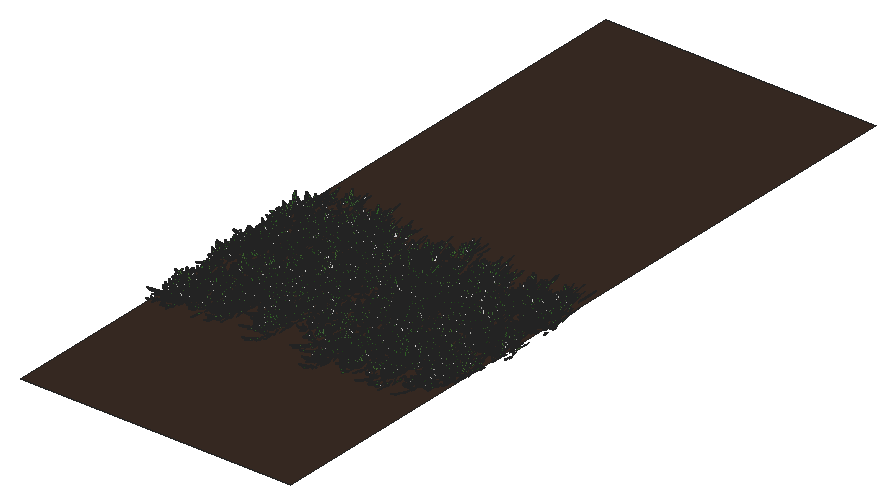
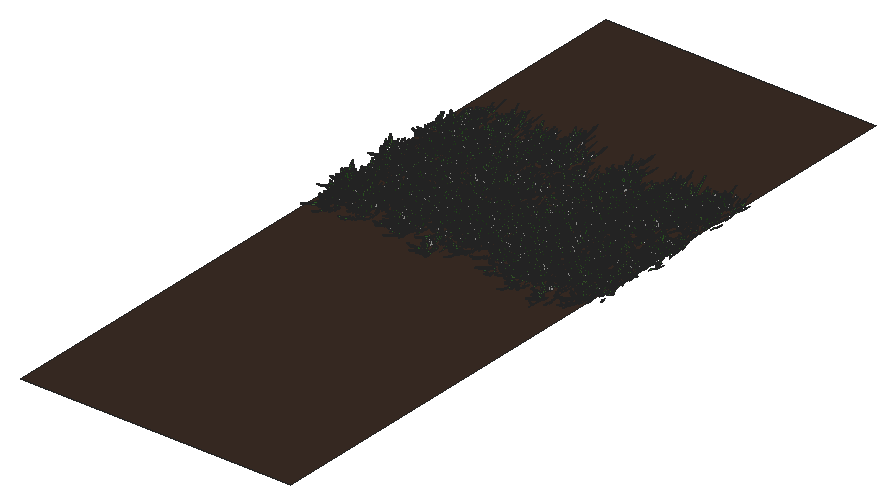
# SketchUp Ruby script. Lengths in inches.
U = 1.inch
M = Sketchup.active_model
def pt(a) = Geom::Point3d.new(a.map { |v| v * U })
def face(e, loops, mat)
  f = e.add_face(loops[0].map { |a| pt(a) })
  loops[1..].each { |l| e.add_face(l.map { |a| pt(a) }).erase! }
  f.material = f.back_material = mat if mat
  f
end
# faces: each face lists its corners as indices into pts; further lists are holes
def faces(e, pts, list, mat = nil) = list.each { |f| face(e, (f[0].is_a?(Array) ? f : [f]).map { |l| l.map { |i| pts[i] } }, mat) }
# xy, xz, yz: faces in a plane at the given z, y or x. An outline is a flat list of corners, or four numbers for a rectangle; further outlines are holes
def ring(l) = l.size == 4 ? [[l[0], l[1]], [l[2], l[1]], [l[2], l[3]], [l[0], l[3]]] : l.each_slice(2).to_a
def flat(e, list, mat, &to3) = list.each { |f| face(e, (f[0].is_a?(Array) ? f : [f]).map { |l| ring(l).map { |u, v| to3.(u, v) } }, mat) }
def xy(e, z, list, mat = nil) = flat(e, list, mat) { |x, y| [x, y, z] }
def xz(e, y, list, mat = nil) = flat(e, list, mat) { |x, z| [x, y, z] }
def yz(e, x, list, mat = nil) = flat(e, list, mat) { |y, z| [x, y, z] }
def lines(e, pts, list) = list.each { |a, b| e.add_line(pt(pts[a]), pt(pts[b])) }
# prism: a flat outline (further loops are holes) pulled along v
def prism(e, loops, v, mat = nil)
  f = face(e, loops, mat); d = Geom::Vector3d.new(v.map { |x| x * U })
  f.pushpull(f.normal.samedirection?(d) ? d.length : -d.length)
end
def box(e, o, s, mat = nil) = prism(e, [[o, [o[0] + s[0], o[1], o[2]], [o[0] + s[0], o[1] + s[1], o[2]], [o[0], o[1] + s[1], o[2]]]], [0, 0, s[2]], mat)
def at(x, y, z, deg = 0) = Geom::Transformation.translation(pt([x, y, z])) * Geom::Transformation.rotation(ORIGIN, Z_AXIS, deg.degrees)
def axes(o, x, y, z) = Geom::Transformation.new([*x, 0, *y, 0, *z, 0, *pt(o).to_a, 1])
def part(name) = M.definitions.add(name)
# library, detail: a bought-in or finely detailed component or shape, given as its bounding box
def library(name, o, s) = part(name).tap { |d| box(d.entities, o, s) }
def detail(e, o, s) = box(e.add_group.entities, o, s)
def put(e, d, t, mat = nil) = e.add_instance(d, t).tap { |i| i.material = mat if mat }
def group(e, t, mat = nil) = e.add_group.tap { |g| g.transformation = t; g.material = mat if mat }.entities
root = M.entities
M.materials.add("Material10").color = [48, 90, 38]
M.materials.add("Material11").color = [68, 110, 48]
M.materials.add("Material12").color = [48, 90, 48]
M.materials.add("Material13").color = [58, 110, 58]
M.materials.add("Material14").color = [58, 90, 38]
M.materials.add("Material15").color = [68, 100, 58]
M.materials.add("Material16").color = [48, 100, 38]
M.materials.add("Material9").color = [68, 110, 58]
M.materials.add("top-soil").color = [58, 44, 36]
c1 = part("grass00")
p = [[-0.6875,0.15,0],[-0.56,0.08,5.52],[-0.04,0.03,2.76],[0.48,-0.02,0],[0.35,-0.02,5.52],[-0.1,-0.14,5.52],
  [-0.12,0.65,8.37],[-0.42,0.65,8.37]]
faces(c1.entities,p,[[0,1,2,3],[3,2,4],[1,5,2],[5,4,2],[1,6,5],[4,5,6],[7,6,1]])
c2 = part("Group16\#1")
put(c2.entities,c1,axes([1.44,-0.61,-0.01],[0.05352,0.12609,0],[-0.10704,0.04543,0.07239],[0.06664,-0.02828,0.11628]),"Material12")
put(c2.entities,c1,axes([0.76,-0.15,-0.01],[0.04676,0.24062,0],[-0.23162,0.04501,0.06642],[0.0652,-0.01267,0.23595]),"Material9")
put(c2.entities,c1,axes([0.79,0.01,-0.01],[-0.00606,0.34651,0],[-0.34381,-0.00602,0.0432],[0.04319,0.00076,0.34386]))
put(c2.entities,c1,axes([1,0.23,-0.01],[-0.07192,0.31144,0],[-0.28722,-0.06632,0.1236],[0.12043,0.02781,0.29478]),"Material11")
put(c2.entities,c1,axes([1.66,0.77,-0.01],[-0.13828,0.29651,0],[-0.21551,-0.1005,0.22471],[0.20365,0.09498,0.23779]),"Material16")
put(c2.entities,c1,axes([0.6875,0.52,-0.01],[-0.18126,0.24051,0],[-0.22746,-0.17142,0.09788],[0.07817,0.05891,0.28481]),"Material11")
put(c2.entities,c1,axes([0.68,0.78,-0.01],[-0.215,0.18688,0],[-0.12385,-0.14248,0.21334],[0.13995,0.16101,0.18878]),"Material9")
put(c2.entities,c1,axes([0.56,1,-0.01],[-0.13756,0.07624,0],[-0.06159,-0.11112,0.0927],[0.04494,0.08108,0.12705]),"Material11")
put(c2.entities,c1,axes([0.2,0.64,-0.01],[-0.23729,0.07254,0],[-0.05711,-0.18681,0.153],[0.04473,0.14632,0.19535]),"Material16")
put(c2.entities,c1,axes([0.0625,0.72,-0.01],[-0.28874,0.02525,0],[-0.02179,-0.24916,0.14647],[0.01276,0.14591,0.25012]),"Material9")
put(c2.entities,c1,axes([-0.08,0.62,-0.01],[-0.34089,-0.04187,0],[0.03255,-0.26504,0.216],[-0.02633,0.21439,0.26703]),"Material16")
put(c2.entities,c1,axes([-0.34,0.98,-0.01],[-0.14314,-0.0493,0],[0.04397,-0.12769,0.06843],[-0.02228,0.0647,0.13505]),"Material16")
put(c2.entities,c1,axes([-0.87,1.45,-0.01],[-0.23488,-0.14114,0],[0.13761,-0.22901,0.06087],[-0.03135,0.05217,0.26717]))
put(c2.entities,c1,axes([-0.72,0.77,-0.01],[-0.14208,-0.13251,0],[0.07209,-0.0773,0.16301],[-0.11118,0.11922,0.1057]),"Material16")
put(c2.entities,c1,axes([-0.62,0.43,-0.01],[-0.14845,-0.21203,0],[0.18654,-0.13061,0.12304],[-0.10079,0.07057,0.22772]),"Material9")
put(c2.entities,c1,axes([-0.68,0.29,-0.01],[-0.13639,-0.32136,0],[0.31723,-0.13464,0.05579],[-0.05136,0.0218,0.34462]),"Material10")
put(c2.entities,c1,axes([-0.64,0.125,-0.01],[-0.0458,-0.23569,0],[0.22124,-0.043,0.08276],[-0.08124,0.01579,0.22538]),"Material13")
put(c2.entities,c1,axes([-1.6,-0.03,-0.01],[0.00576,-0.32897,0],[0.27526,0.00482,0.18018],[-0.18015,-0.00315,0.2753]),"Material11")
put(c2.entities,c1,axes([-1.36,-0.31,-0.01],[0.05718,-0.24765,0],[0.18172,0.04196,0.17267],[-0.16825,-0.03885,0.1865]),"Material16")
put(c2.entities,c1,axes([-1.54,-0.72,-0.01],[0.06537,-0.14017,0],[0.13555,0.06321,0.03939],[-0.0357,-0.01665,0.14956]))
put(c2.entities,c1,axes([-1.19,-0.9,-0.01],[0.09597,-0.12735,0],[0.11214,0.08451,0.07557],[-0.06035,-0.04548,0.14042]),"Material15")
put(c2.entities,c1,axes([-0.47,-0.54,-0.01],[0.11588,-0.10072,0],[0.0618,0.0711,0.12124],[-0.07953,-0.0915,0.0942]))
put(c2.entities,c1,axes([-0.47,-0.84,-0.01],[0.11927,-0.0661,0],[0.06603,0.11913,0.00646],[-0.00313,-0.00565,0.13621]),"Material11")
put(c2.entities,c1,axes([-0.38,-1.24,-0.01],[0.28037,-0.08571,0],[0.0618,0.20215,0.20315],[-0.05939,-0.19428,0.21139]),"Material15")
put(c2.entities,c1,axes([-0.06,-0.66,-0.01],[0.22719,-0.01987,0],[0.01247,0.14255,0.17758],[-0.01547,-0.17691,0.1431]),"Material14")
put(c2.entities,c1,axes([0.11,-0.89,-0.01],[0.14882,0.01828,0],[-0.01058,0.08611,0.12229],[0.01491,-0.12138,0.08676]),"Material12")
put(c2.entities,c1,axes([0.25,-0.72,-0.01],[0.20481,0.07053,0],[-0.06206,0.18022,0.10291],[0.03351,-0.0973,0.1906]),"Material12")
put(c2.entities,c1,axes([0.85,-1.42,-0.01],[0.16481,0.09904,0],[-0.09472,0.15762,0.05616],[0.02893,-0.04814,0.18389]),"Material11")
put(c2.entities,c1,axes([1.01,-1.09,-0.01],[0.21858,0.20385,0],[-0.17495,0.1876,0.15339],[0.10462,-0.11218,0.25652]),"Material16")
put(c2.entities,c1,axes([1.01,-0.71,-0.01],[0.08733,0.12473,0],[-0.06445,0.04512,0.13037],[0.1068,-0.07477,0.07867]),"Material12")
c3 = part("Group15\#1")
put(c3.entities,c2,at(0,0,0))
c4 = part("3darcstudiotree_grass00\#1")
put(c4.entities,c3,at(0,0,0))
xy(root,12.99,[[800.04,262.41,979.6875,748.39]],"top-soil")
put(root,c4,axes([910.99,376.34,12.99],[0.80476,6.1803,0],[-2.5153,1.71139,-0.00785],[-0.03971,0.02702,1.89978]))
put(root,c4,axes([812.23,382.27,12.99],[2.52246,-5.10895,0],[2.10471,5.42989,-0.01442],[0.04193,0.10816,1.90876]))
put(root,c4,axes([950.38,381.34,12.99],[1.57393,4.5753,0],[-2.62689,4.72186,-0.01217],[-0.03801,0.06833,1.82194]))
put(root,c4,axes([803.39,383.91,12.99],[2.02408,-5.39153,0],[2.64381,5.18621,-0.00643],[0.01727,0.03388,1.6911]))
put(root,c4,axes([943.31,384.47,12.99],[3.24773,-0.60424,0],[0.26081,7.32474,-0.02372],[0.00647,0.18181,1.48337]))
put(root,c4,axes([870.54,382.84,12.99],[1.30187,6.81409,0],[-2.51328,2.50904,-0.01938],[-0.07503,0.0749,1.58937]))
put(root,c4,axes([910.61,382.43,12.99],[-2.5691,-1.45972,0],[0.80318,-7.38629,-0.01735],[0.01559,-0.14339,1.70162]))
put(root,c4,axes([807.77,382.39,12.99],[-2.25937,3.85947,0],[-1.45949,-4.46443,-0.01872],[-0.05442,-0.16647,1.62421]))
put(root,c4,axes([816.375,386.45,12.99],[1.10174,-5.55163,0],[2.97048,3.08028,-0.00454],[0.01203,0.01247,1.30224]))
put(root,c4,axes([827.21,386.19,12.99],[0.08987,-6.94735,0],[3.24927,0.21962,-0.0158],[0.06108,0.00413,1.72451]))
put(root,c4,axes([838.09,385.71,12.99],[-0.77245,-5.44279,0],[3.02945,-2.24655,-0.01227],[0.04916,-0.03645,1.83962]))
put(root,c4,axes([841.9,385.69,12.99],[1.64248,5.29002,0],[-2.43182,3.94529,-0.0048],[-0.01519,0.02464,1.58899]))
put(root,c4,axes([965.05,386.93,12.99],[-1.33501,-5.28345,0],[2.34355,-3.09418,-0.00817],[0.02964,-0.03913,1.55447]))
put(root,c4,axes([929.3,385.85,12.99],[-1.89685,5.08823,0],[-2.49499,-4.86003,-0.01912],[-0.04377,-0.08527,1.35238]))
put(root,c4,axes([923.76,386.65,12.99],[-2.62192,3.16233,0],[-1.33999,-5.80523,-0.01893],[-0.03076,-0.13327,1.37131]))
put(root,c4,axes([865.75,389.8,12.99],[-3.05838,-2.89505,0],[0.97921,-5.40527,-0.00358],[0.00645,-0.03563,1.65637]))
put(root,c4,axes([831.47,392.35,12.99],[2.93383,-2.52255,0],[0.98457,5.98339,-0.01237],[0.02098,0.12751,1.84855]))
put(root,c4,axes([809,393.23,12.99],[0.59751,-5.96003,0],[2.8542,1.49516,-0.01662],[0.07313,0.03831,1.81323]))
put(root,c4,axes([905.28,392.21,12.99],[-2.7394,-4.27584,0],[1.38803,-4.64665,-0.01838],[0.05553,-0.1859,1.80866]))
put(root,c4,axes([820.61,394.35,12.99],[3.47703,-0.80176,0],[0.32671,7.40353,-0.01121],[0.0033,0.07467,1.30781]))
put(root,c4,axes([814.98,391.37,12.99],[-2.59581,-0.64838,0],[0.36498,-7.63528,-0.01667],[0.00703,-0.14714,1.79039]))
put(root,c4,axes([895.36,393.09,12.99],[1.4896,7.10078,0],[-2.62457,2.87692,-0.00104],[-0.0037,0.00405,1.58037]))
put(root,c4,axes([839.95,395.5,12.99],[2.05349,3.10989,0],[-1.87462,6.46795,-0.00365],[-0.00583,0.02012,1.34685]))
put(root,c4,axes([926.77,396.61,12.99],[2.91866,-2.95139,0],[1.07373,5.54825,-0.00969],[0.01465,0.07569,1.36001]))
put(root,c4,axes([970.2,394.14,12.99],[-3.10367,0.52847,0],[-0.19217,-5.8972,-0.0204],[-0.00584,-0.17916,1.3669]))
put(root,c4,axes([917.19,395.15,12.99],[-2.70392,-3.68343,0],[1.4747,-5.65654,-0.01663],[0.04193,-0.16083,1.94585]))
put(root,c4,axes([862.23,395.05,12.99],[-2.00461,4.44894,0],[-2.20387,-5.18878,-0.01854],[-0.053,-0.12479,1.78092]))
put(root,c4,axes([964.49,399.41,12.99],[2.75356,-2.67524,0],[1.28145,6.8919,-0.00549],[0.00688,0.03702,1.44062]))
put(root,c4,axes([947.2,396.12,12.99],[-1.59665,6.45122,0],[-2.59665,-3.35805,-0.02589],[-0.07716,-0.09979,1.40149]))
put(root,c4,axes([967.09,396.55,12.99],[-2.2526,3.80773,0],[-1.77986,-5.50186,-0.01371],[-0.02607,-0.08059,1.31321]))
put(root,c4,axes([856.66,400.25,12.99],[2.50921,-2.51893,0],[1.2451,6.48083,-0.00525],[0.0082,0.04267,1.64886]))
put(root,c4,axes([837,400.07,12.99],[2.47061,0.56833,0],[-0.31846,7.23386,-0.00091],[-0.00031,0.00694,1.45853]))
put(root,c4,axes([949.79,399.66,12.99],[-1.80261,-6.14006,0],[2.27121,-3.48411,-0.00883],[0.0372,-0.05707,1.90461]))
put(root,c4,axes([906.43,398.99,12.99],[-0.90926,6.89194,0],[-2.75226,-1.89733,-0.01363],[-0.04678,-0.03225,1.41312]))
put(root,c4,axes([869.82,401.1,12.99],[-0.98905,-5.60811,0],[2.66514,-2.45598,-0.00075],[0.00269,-0.00248,1.52674]))
put(root,c4,axes([939.73,400.57,12.99],[-2.06296,-2.94287,0],[1.62821,-5.96396,-0.00523],[0.01222,-0.04477,1.86317]))
put(root,c4,axes([919.09,400.7,12.99],[-2.97965,-1.14436,0],[0.45554,-6.19771,-0.01654],[0.01379,-0.18758,1.89711]))
put(root,c4,axes([820.05,401.16,12.99],[-2.39735,-2.64179,0],[1.08722,-5.15535,-0.00927],[0.02336,-0.11076,1.99366]))
put(root,c4,axes([812.34,400.85,12.99],[-2.17098,-2.55399,0],[1.5691,-6.96936,-0.00712],[0.01141,-0.05069,1.64666]))
put(root,c4,axes([884.61,403.71,12.99],[0.71077,-5.96983,0],[2.44818,1.52307,-0.01758],[0.08367,0.05205,1.71636]))
put(root,c4,axes([803.41,401.87,12.99],[-2.65714,1.91919,0],[-0.86351,-6.24695,-0.02199],[-0.02536,-0.18349,1.50537]))
put(root,c4,axes([898.16,404.375,12.99],[-1.40162,-6.52875,0],[2.73423,-3.0672,-0.01008],[0.0339,-0.03803,1.566]))
put(root,c4,axes([845.53,404.56,12.99],[-1.63209,-6.76231,0],[2.79431,-3.52394,-0.0117],[0.04012,-0.05059,1.7149]))
put(root,c4,axes([817.48,405.46,12.99],[2.07451,3.88446,0],[-1.55934,4.35143,-0.00694],[-0.02077,0.05795,1.5947]))
put(root,c4,axes([975.38,405.87,12.99],[0.67244,7.51516,0],[-2.8226,1.31968,-0.01369],[-0.04759,0.02225,1.40267]))
put(root,c4,axes([873.32,410.7,12.99],[-0.50031,-7.24226,0],[3.08195,-1.11249,-0.01303],[0.05922,-0.02138,1.96953]))
put(root,c4,axes([917.66,409.17,12.99],[0.44995,6.15696,0],[-2.49999,0.95465,-0.00028],[-0.00121,0.00046,1.50491]))
put(root,c4,axes([934.8125,411.9,12.99],[2.73922,-1.83439,0],[0.85135,6.6428,-0.01036],[0.01357,0.10587,1.93559]))
put(root,c4,axes([849.78,411.43,12.99],[-2.43074,-3.16588,0],[1.29079,-5.17852,-0.01205],[0.02223,-0.08917,1.33255]))
put(root,c4,axes([967.03,410.42,12.99],[-1.6235,5.69663,0],[-2.93452,-4.36995,-0.00953],[-0.02454,-0.03654,1.47621]))
put(root,c4,axes([925.7,412.05,12.99],[-2.25924,-2.71771,0],[1.25782,-5.46367,-0.01604],[0.03835,-0.16659,1.9024]))
put(root,c4,axes([950.58,411.35,12.99],[-1.11464,6.3418,0],[-2.79983,-2.57133,-0.02547],[-0.07915,-0.07269,1.38631]))
put(root,c4,axes([860.21,414.98,12.99],[1.71225,-6.25716,0],[2.7276,3.90009,-0.01393],[0.0387,0.05534,1.44657]))
put(root,c4,axes([954.98,413.42,12.99],[-2.04299,-5.58205,0],[2.31505,-4.42729,-0.01878],[0.05849,-0.11185,1.68146]))
put(root,c4,axes([852.1,414.07,12.99],[3.10859,2.98565,0],[-1.09536,5.95917,-0.00848],[-0.01621,0.08819,1.91304]))
put(root,c4,axes([833,414.5,12.99],[-1.16298,-6.58233,0],[2.81309,-2.59706,-0.01424],[0.04553,-0.04203,1.43479]))
put(root,c4,axes([964.71,413.78,12.99],[-2.49087,-4.37206,0],[1.80532,-5.37433,-0.00705],[0.0194,-0.05776,1.8369]))
put(root,c4,axes([975.45,412.56,12.99],[-1.84084,5.67397,0],[-2.36228,-4.00466,-0.0152],[-0.03997,-0.06776,1.3203]))
put(root,c4,axes([840.79,413.81,12.99],[-2.47244,-0.67361,0],[0.35958,-6.89641,-0.01308],[0.00611,-0.11717,1.64432]))
put(root,c4,axes([947.97,415.13,12.99],[-2.31036,-4.02201,0],[1.74332,-5.2326,-0.01582],[0.03337,-0.10018,1.37394]))
put(root,c4,axes([886.09,413.84,12.99],[-2.61204,2.96858,0],[-1.31678,-6.05412,-0.01143],[-0.01697,-0.07803,1.35283]))
put(root,c4,axes([835.46,415.25,12.99],[-2.7337,-4.78902,0],[1.98127,-5.90954,-0.01589],[0.03002,-0.08955,1.38765]))
put(root,c4,axes([927.84,419.89,12.99],[3.41586,-0.06235,0],[0.02574,7.3693,-0.00522],[0.00013,0.03859,1.42947]))
put(root,c4,axes([941.78,419.93,12.99],[0.49895,-7.73961,0],[3.0917,1.04145,-0.00777],[0.02426,0.00817,1.3523]))
put(root,c4,axes([851.91,420.33,12.99],[2.9374,-0.01843,0],[0.00857,7.13781,-0.02008],[0.00021,0.17317,1.61638]))
put(root,c4,axes([845.18,420.31,12.99],[-0.55708,-6.57859,0],[2.39989,-1.06189,-0.00678],[0.03065,-0.01356,1.54322]))
put(root,c4,axes([818.97,421.5,12.99],[2.41044,-3.97435,0],[1.78683,5.66265,-0.00659],[0.01801,0.05706,1.95827]))
put(root,c4,axes([824.61,421.31,12.99],[2.93575,-0.57171,0],[0.22452,6.0242,-0.01096],[0.00496,0.1332,1.93666]))
put(root,c4,axes([922.6875,421.48,12.99],[3.10965,3.61865,0],[-1.54408,6.93329,-0.01612],[-0.02537,0.11393,1.61949]))
put(root,c4,axes([906.27,422.89,12.99],[3.10471,-0.57753,0],[0.2459,6.90744,-0.01977],[0.00616,0.17316,1.59866]))
put(root,c4,axes([877.13,423.71,12.99],[2.55397,-1.14656,0],[0.54623,6.35774,-0.00241],[0.00213,0.02485,1.79003]))
put(root,c4,axes([869.64,421.6,12.99],[-0.52743,6.70127,0],[-3.0663,-1.26104,-0.02584],[-0.07747,-0.03186,1.30174]))
put(root,c4,axes([839.51,421.92,12.99],[-0.1939,7.89486,0],[-2.44434,-0.31369,-0.00552],[-0.02419,-0.0031,1.47331]))
put(root,c4,axes([890.85,422.43,12.99],[-0.62515,5.72474,0],[-2.659,-1.51723,-0.00012],[-0.00042,-0.00024,1.39497]))
put(root,c4,axes([926.41,427.23,12.99],[0.30994,-6.26719,0],[3.45198,0.89203,-0.01256],[0.04998,0.01291,1.90836]))
put(root,c4,axes([856.78,428.08,12.99],[2.43953,-2.95496,0],[1.52618,6.58363,-0.00115],[0.00171,0.00739,1.42878]))
put(root,c4,axes([959.625,428.39,12.99],[2.94744,0.50852,0],[-0.25673,7.77514,-0.00004],[-0.00001,0.00039,1.93334]))
put(root,c4,axes([962.72,429.39,12.99],[3.19852,2.38704,0],[-1.01104,7.07883,-0.00124],[-0.00142,0.00994,1.65228]))
put(root,c4,axes([801.1,430.27,12.99],[2.45511,-0.83044,0],[0.48099,7.43033,-0.00326],[0.002,0.03092,1.88794]))
put(root,c4,axes([833.44,427.09,12.99],[-2.56611,-1.3902,0],[0.80604,-7.77423,-0.00987],[0.00705,-0.06799,1.48448]))
put(root,c4,axes([919.38,428.89,12.99],[-1.20969,-5.54324,0],[2.5053,-2.85677,-0.00448],[0.01995,-0.02275,1.90991]))
put(root,c4,axes([840.89,429.72,12.99],[2.37945,5.1381,0],[-2.38882,5.78048,-0.01632],[-0.03438,0.0832,1.46423]))
put(root,c4,axes([896.8125,430.44,12.99],[-1.77128,-4.16863,0],[1.93043,-4.286,-0.02073],[0.06241,-0.13857,1.5494]))
put(root,c4,axes([940.11,431.69,12.99],[2.52204,0.17989,0],[-0.08167,5.98301,-0.01718],[-0.00281,0.20554,1.88076]))
put(root,c4,axes([827.27,432.32,12.99],[2.47937,-2.70783,0],[1.19152,5.70067,-0.01719],[0.03331,0.15936,1.70421]))
put(root,c4,axes([946.44,429.49,12.99],[-2.27029,5.27019,0],[-2.14493,-4.82808,-0.02428],[-0.05568,-0.12533,1.32917]))
put(root,c4,axes([907.21,429.73,12.99],[-3.33796,1.47306,0],[-0.55537,-6.57587,-0.00152],[-0.00101,-0.01201,1.41339]))
put(root,c4,axes([851.66,432.63,12.99],[0.2778,-5.70209,0],[2.99615,0.76271,-0.00391],[0.01311,0.00334,1.39627]))
put(root,c4,axes([805.02,433.82,12.99],[1.98027,-6.08525,0],[2.78088,4.72861,-0.01386],[0.03054,0.05194,1.30579]))
put(root,c4,axes([869.44,433.72,12.99],[2.58549,-5.04669,0],[1.73104,4.63392,-0.01134],[0.03037,0.0813,1.5074]))
put(root,c4,axes([898.38,436.74,12.99],[1.08769,-5.68165,0],[2.23177,2.23247,-0.00213],[0.00762,0.00762,1.30651]))
put(root,c4,axes([870.93,437.13,12.99],[2.59343,-2.38882,0],[0.92889,5.26939,-0.02314],[0.03411,0.1935,1.34449]))
put(root,c4,axes([839.24,437.32,12.99],[2.36138,-2.55413,0],[1.08274,5.23059,-0.01286],[0.02313,0.11173,1.45976]))
put(root,c4,axes([962.35,437.98,12.99],[2.63347,-4.05177,0],[1.38258,4.69546,-0.0013],[0.00319,0.01083,1.49257]))
put(root,c4,axes([901.59,437.73,12.99],[1.57463,4.71078,0],[-2.28322,3.98784,-0.0123],[-0.03965,0.06926,1.59876]))
put(root,c4,axes([847.8,436.51,12.99],[-2.05969,4.64081,0],[-2.25266,-5.22408,-0.00446],[-0.0103,-0.02388,1.44777]))
put(root,c4,axes([815.64,438.23,12.99],[0.79553,5.55248,0],[-2.74879,2.05785,-0.00037],[-0.00123,0.00092,1.37352]))
put(root,c4,axes([922.32,440.875,12.99],[2.82273,-2.30568,0],[1.04177,6.66417,-0.0155],[0.02454,0.157,1.9985]))
put(root,c4,axes([906.66,437.61,12.99],[-2.80439,4.11231,0],[-1.58808,-5.65887,-0.01729],[-0.0377,-0.13434,1.62898]))
put(root,c4,axes([971.78,439.82,12.99],[-1.51264,-4.5175,0],[2.29442,-4.01434,-0.02737],[0.07139,-0.1249,1.30175]))
put(root,c4,axes([948.62,439.6875,12.99],[-3.36819,1.28778,0],[-0.53926,-7.36978,-0.00717],[-0.00397,-0.05432,1.50735]))
put(root,c4,axes([800.21,442.51,12.99],[2.40908,2.98899,0],[-1.50869,6.35379,-0.01651],[-0.03287,0.13845,1.81134]))
put(root,c4,axes([864.47,440.67,12.99],[-3.16063,-0.04144,0],[0.01457,-5.80642,-0.00073],[0.00002,-0.0072,1.50826]))
put(root,c4,axes([914.55,442,12.99],[-2.30767,-5.00508,0],[2.10075,-5.06106,-0.00166],[0.00475,-0.01145,1.74215]))
put(root,c4,axes([804.59,441.83,12.99],[-2.59166,1.48168,0],[-0.64564,-5.90089,-0.00789],[-0.00903,-0.08254,1.7222]))
put(root,c4,axes([979.11,442.07,12.99],[-2.95008,3.6636,0],[-1.24769,-5.24975,-0.00649],[-0.01228,-0.05165,1.42064]))
put(root,c4,axes([937.48,446.02,12.99],[-1.07774,-6.16599,0],[2.30064,-2.1012,-0.01431],[0.06792,-0.06203,1.73701]))
put(root,c4,axes([870.49,447.21,12.99],[1.47021,-4.84525,0],[2.88108,4.56797,-0.02169],[0.05833,0.09248,1.57389]))
put(root,c4,axes([975.17,446.33,12.99],[1.53323,4.6828,0],[-2.32061,3.97017,-0.0157],[-0.05083,0.08697,1.60759]))
put(root,c4,axes([853.26,448.74,12.99],[1.72826,-5.44789,0],[2.55308,4.23203,-0.00976],[0.03459,0.05734,1.89325]))
put(root,c4,axes([804.14,448.51,12.99],[2.35891,4.38091,0],[-1.68949,4.75343,-0.0068],[-0.01618,0.04552,1.38619]))
put(root,c4,axes([893.79,449.77,12.99],[-0.17442,-7.312,0],[2.45442,-0.30592,-0.01049],[0.04564,-0.00569,1.4693]))
put(root,c4,axes([963.02,448.55,12.99],[0.75222,5.89541,0],[-3.15272,2.10194,-0.00405],[-0.01169,0.0078,1.35389]))
put(root,c4,axes([913.9375,450.31,12.99],[1.82097,3.71376,0],[-1.71334,4.38974,-0.00625],[-0.02037,0.0522,1.72796]))
put(root,c4,axes([827.03,451.67,12.99],[2.54894,-1.15241,0],[0.49169,5.68257,-0.00259],[0.00245,0.02837,1.70099]))
put(root,c4,axes([943.25,451.5,12.99],[-0.03522,-6.11651,0],[3.32991,-0.10018,-0.00745],[0.03167,-0.00095,1.94284]))
put(root,c4,axes([884.67,449.9375,12.99],[0.10005,5.82927,0],[-3.06221,0.27463,-0.00595],[-0.02803,0.00251,1.98232]))
put(root,c4,axes([898.48,449.36,12.99],[-2.13663,6.17743,0],[-2.14771,-3.88152,-0.0043],[-0.01683,-0.03042,1.8735]))
put(root,c4,axes([855.85,449.51,12.99],[-2.35339,3.98124,0],[-1.8417,-5.68851,-0.01624],[-0.04144,-0.128,1.82169]))
put(root,c4,axes([959.41,450.1,12.99],[-1.75527,5.56067,0],[-2.01976,-3.33135,-0.00844],[-0.02829,-0.04667,1.41311]))
put(root,c4,axes([949.98,452.24,12.99],[-3.01598,0.47779,0],[-0.16876,-5.56642,-0.01842],[-0.00513,-0.16909,1.34789]))
put(root,c4,axes([933.73,452.5,12.99],[-3.02212,-2.07398,0],[0.92072,-7.01031,-0.01736],[0.0152,-0.1157,1.33702]))
put(root,c4,axes([878.11,452.69,12.99],[-3.02101,-2.61547,0],[1.20407,-7.26707,-0.00084],[0.00085,-0.00515,1.34285]))
put(root,c4,axes([872.57,455.59,12.99],[1.2352,-7.44457,0],[2.29503,1.9897,-0.00605],[0.03282,0.02845,1.95327]))
put(root,c4,axes([840.55,456.55,12.99],[3.11387,1.27941,0],[-0.55883,7.10689,-0.00017],[-0.00013,0.0016,1.78268]))
put(root,c4,axes([823.79,456.67,12.99],[2.79179,1.19408,0],[-0.5102,6.23291,-0.00485],[-0.00412,0.05028,1.75633]))
put(root,c4,axes([817.18,456.95,12.99],[-0.2876,-5.58913,0],[2.69209,-0.72383,-0.01277],[0.04715,-0.01268,1.38207]))
put(root,c4,axes([970.36,456.38,12.99],[-2.16259,-6.31541,0],[2.68465,-4.80359,-0.01534],[0.04446,-0.07956,1.72134]))
put(root,c4,axes([837.76,458.99,12.99],[1.03781,-5.69119,0],[2.70702,2.57934,-0.02113],[0.07347,0.07,1.51549]))
put(root,c4,axes([901.84,457.5625,12.99],[-2.06551,-3.0211,0],[1.31335,-4.69188,-0.02395],[0.05387,-0.19246,1.39534]))
put(root,c4,axes([955.72,457.89,12.99],[1.63233,6.19412,0],[-3.00587,4.13907,-0.01693],[-0.0482,0.06638,1.59984]))
put(root,c4,axes([864.61,456.83,12.99],[-2.54121,2.43966,0],[-1.07909,-5.87319,-0.01995],[-0.0328,-0.1785,1.62326]))
put(root,c4,axes([808.42,457.7,12.99],[-3.0442,0.27099,0],[-0.09606,-5.63869,-0.00954],[-0.00155,-0.09101,1.41434]))
put(root,c4,axes([846.09,457.73,12.99],[-1.67231,4.72703,0],[-1.98511,-3.6696,-0.00747],[-0.02246,-0.04152,1.35493]))
put(root,c4,axes([905.3,461.18,12.99],[0.07267,-5.98865,0],[2.63732,0.16721,-0.00183],[0.00748,0.00047,1.48199]))
put(root,c4,axes([802.55,459.13,12.99],[-3.48726,0.58337,0],[-0.23034,-7.19455,-0.0067],[-0.00148,-0.0462,1.30916]))
put(root,c4,axes([889.35,461.91,12.99],[3.01111,2.47643,0],[-0.87267,5.54444,-0.01256],[-0.0219,0.13913,1.82155]))
put(root,c4,axes([947.67,460.38,12.99],[-2.8082,4.4927,0],[-1.57679,-5.14992,-0.01309],[-0.03737,-0.12204,1.87779]))
put(root,c4,axes([917.65,461.76,12.99],[0.3609,6.80773,0],[-3.37531,0.935,-0.01569],[-0.04962,0.01374,1.48562]))
put(root,c4,axes([920.04,465.8,12.99],[2.85908,2.23845,0],[-0.8407,5.6108,-0.02009],[-0.03193,0.21312,1.7458]))
put(root,c4,axes([813.27,466.83,12.99],[0.54088,-7.28857,0],[3.31922,1.28706,-0.00997],[0.03159,0.01225,1.48373]))
put(root,c4,axes([927.39,464.48,12.99],[-0.96063,5.32352,0],[-2.68448,-2.53118,-0.01866],[-0.0674,-0.06356,1.55626]))
put(root,c4,axes([802.89,467.74,12.99],[0.80159,-6.28447,0],[2.57551,1.71653,-0.01207],[0.05237,0.03491,1.66287]))
put(root,c4,axes([825.48,466.29,12.99],[2.07888,5.77278,0],[-2.07902,3.91208,-0.01155],[-0.04098,0.0771,1.69697]))
put(root,c4,axes([922.9375,466.49,12.99],[-2.10374,-4.21424,0],[1.68632,-4.39864,-0.01406],[0.04683,-0.12215,1.77353]))
put(root,c4,axes([889.96,469.15,12.99],[1.84942,-3.73329,0],[1.72186,4.45706,-0.01409],[0.04297,0.11123,1.64399]))
put(root,c4,axes([971.61,469.9,12.99],[1.26594,-5.58778,0],[2.61227,3.09242,-0.01075],[0.03522,0.0417,1.48923]))
put(root,c4,axes([950.56,470.29,12.99],[2.96237,-3.27223,0],[1.30935,6.1938,-0.00312],[0.00572,0.02704,1.73901]))
put(root,c4,axes([840.87,466.85,12.99],[-2.9933,0.23282,0],[-0.11174,-7.50665,-0.01213],[-0.00171,-0.11475,1.86653]))
put(root,c4,axes([898.68,470.5,12.99],[3.41008,-0.52285,0],[0.22554,7.68634,-0.00473],[0.00102,0.03492,1.49489]))
put(root,c4,axes([856.42,467.3125,12.99],[-1.51012,6.35316,0],[-2.77066,-3.4412,-0.0267],[-0.07147,-0.08876,1.31753]))
put(root,c4,axes([909.8,469.41,12.99],[-1.94109,-6.21668,0],[2.53159,-4.13034,-0.01802],[0.04625,-0.07546,1.345]))
put(root,c4,axes([863.89,470.6,12.99],[2.68227,1.50181,0],[-0.82745,7.72209,-0.01455],[-0.01436,0.134,1.97892]))
put(root,c4,axes([930.67,467.93,12.99],[-0.88224,7.091,0],[-2.67796,-1.74096,-0.01558],[-0.07461,-0.0485,1.90128]))
put(root,c4,axes([946.56,469.72,12.99],[-2.78447,-3.55245,0],[1.6793,-6.87775,-0.0179],[0.03005,-0.12308,1.62858]))
put(root,c4,axes([894.35,474.24,12.99],[3.02159,2.19078,0],[-0.92181,6.64327,-0.00141],[-0.00199,0.01435,1.95289]))
put(root,c4,axes([856.85,475.14,12.99],[0.58056,-6.28383,0],[2.71707,1.31169,-0.00249],[0.01005,0.00485,1.57305]))
put(root,c4,axes([930.13,475.32,12.99],[0.60188,-5.74686,0],[2.69504,1.47486,-0.00366],[0.01418,0.00776,1.51551]))
put(root,c4,axes([935.36,475.6875,12.99],[3.33852,-0.7301,0],[0.24996,5.97237,-0.00501],[0.00215,0.05142,1.62495]))
put(root,c4,axes([877.1,476.24,12.99],[0.24638,-7.23344,0],[2.84276,0.50594,-0.01871],[0.08558,0.01523,1.79426]))
put(root,c4,axes([839.99,474.64,12.99],[-1.91113,-3.66316,0],[2.07333,-5.65208,-0.0116],[0.02361,-0.06436,1.40225]))
put(root,c4,axes([913.2,474.03,12.99],[-0.18999,6.45208,0],[-3.27716,-0.50423,-0.01753],[-0.07294,-0.01122,1.87889]))
put(root,c4,axes([882.56,476.96,12.99],[2.34571,-2.14303,0],[1.23215,7.04715,-0.02256],[0.02867,0.16398,1.55958]))
put(root,c4,axes([824.01,474.23,12.99],[-2.5521,1.18349,0],[-0.53357,-6.01214,-0.01756],[-0.01676,-0.18881,1.76676]))
put(root,c4,axes([979.03,477.22,12.99],[1.15371,-5.21123,0],[2.59817,3.0056,-0.00728],[0.02165,0.02504,1.33141]))
put(root,c4,axes([907.7,476.79,12.99],[2.56018,2.49977,0],[-1.19164,6.37705,-0.00364],[-0.00674,0.03604,1.96053]))
put(root,c4,axes([853.22,474.81,12.99],[-2.4648,-1.01261,0],[0.52278,-6.64913,-0.01818],[0.01073,-0.13643,1.35222]))
put(root,c4,axes([802.88,475.78,12.99],[-0.28607,6.77517,0],[-3.48193,-0.7682,-0.01578],[-0.04486,-0.0099,1.37044]))
put(root,c4,axes([970.48,476.41,12.99],[-2.95742,-2.48444,0],[0.94503,-5.87811,-0.00277],[0.00351,-0.02181,1.38049]))
put(root,c4,axes([939.47,476.3,12.99],[-2.28252,-2.28686,0],[1.32136,-6.89132,-0.00176],[0.00306,-0.01594,1.95594]))
put(root,c4,axes([966.72,479.87,12.99],[2.47022,-0.05925,0],[0.02999,6.53205,-0.01029],[0.00038,0.08334,1.389]))
put(root,c4,axes([861.63,479.29,12.99],[-1.20509,-7.41793,0],[3.04519,-2.58497,-0.00006],[0.00024,-0.0002,1.81412]))
put(root,c4,axes([950.07,478.61,12.99],[-1.99297,-5.03238,0],[2.43328,-5.0353,-0.01753],[0.04273,-0.08843,1.48083]))
put(root,c4,axes([976.05,479.36,12.99],[2.84812,3.08729,0],[-1.05217,5.07193,-0.0026],[-0.006,0.02891,1.81639]))
put(root,c4,axes([818.89,477.95,12.99],[-2.3513,-1.75058,0],[1.00093,-7.02485,-0.00123],[0.00168,-0.0118,1.95221]))
put(root,c4,axes([898.07,478.41,12.99],[-3.25805,1.56903,0],[-0.59781,-6.48631,-0.00142],[-0.0012,-0.01298,1.63114]))
put(root,c4,axes([828.22,479.36,12.99],[-2.65853,-1.91192,0],[0.92532,-6.72313,-0.00258],[0.00247,-0.01798,1.35273]))
put(root,c4,axes([886.07,478.89,12.99],[-2.78952,4.68743,0],[-1.5177,-4.71938,-0.00523],[-0.01297,-0.04034,1.47184]))
put(root,c4,axes([918.06,484,12.99],[1.5568,-6.56755,0],[2.62898,3.25627,-0.00988],[0.03998,0.04952,1.88737]))
put(root,c4,axes([866.8,484.76,12.99],[2.56908,-2.40603,0],[0.96449,5.38118,-0.00746],[0.01238,0.06906,1.52751]))
put(root,c4,axes([848.87,484.36,12.99],[-1.29031,-6.17304,0],[2.92616,-3.19593,-0.00689],[0.02435,-0.0266,1.74288]))
put(root,c4,axes([972.15,485.17,12.99],[1.93397,3.689,0],[-1.60567,4.39846,-0.00812],[-0.02444,0.06696,1.6158]))
put(root,c4,axes([816.55,483.625,12.99],[-2.56775,2.06083,0],[-0.90778,-5.91011,-0.01418],[-0.02268,-0.14766,1.8149]))
put(root,c4,axes([870.32,485.83,12.99],[-1.46361,-7.17062,0],[2.86098,-3.05132,-0.01753],[0.05496,-0.05862,1.49864]))
put(root,c4,axes([884.25,484.21,12.99],[-0.78907,6.12371,0],[-2.86591,-1.92959,-0.01201],[-0.04106,-0.02764,1.46096]))
put(root,c4,axes([934.14,487.29,12.99],[0.18924,-6.87998,0],[2.78345,0.40005,-0.00515],[0.02355,0.00338,1.75106]))
put(root,c4,axes([952.14,484.73,12.99],[-2.77419,0.34926,0],[-0.17417,-7.22889,-0.02509],[-0.00428,-0.17745,1.34616]))
put(root,c4,axes([906.49,487,12.99],[1.99817,3.98355,0],[-2.2895,6.00076,-0.01764],[-0.04238,0.11107,1.74631]))
put(root,c4,axes([963.09,488.07,12.99],[2.97302,-1.38054,0],[0.50797,5.71595,-0.00331],[0.00299,0.03366,1.58887]))
put(root,c4,axes([881.51,488.3,12.99],[-0.70817,-6.56092,0],[2.54682,-1.43641,-0.01268],[0.05494,-0.03099,1.60602]))
put(root,c4,axes([851.88,488.94,12.99],[0.23898,-6.90862,0],[2.73702,0.49471,-0.00365],[0.01491,0.0027,1.54435]))
put(root,c4,axes([844.58,486.39,12.99],[-2.75522,3.47475,0],[-1.36718,-5.6645,-0.01481],[-0.02646,-0.10963,1.43556]))
put(root,c4,axes([958.66,486.66,12.99],[-1.85089,3.96583,0],[-2.22457,-5.42499,-0.02311],[-0.04913,-0.11981,1.38694]))
put(root,c4,axes([800.7,486.62,12.99],[-1.59854,6.27157,0],[-2.9046,-3.86847,-0.00219],[-0.00675,-0.00899,1.64693]))
put(root,c4,axes([822.93,487.01,12.99],[-1.67603,4.05622,0],[-2.41079,-5.20503,-0.01576],[-0.04724,-0.10199,1.87507]))
put(root,c4,axes([926.63,487.29,12.99],[-3.23346,2.99993,0],[-1.15398,-6.49923,-0.01879],[-0.02467,-0.13896,1.46955]))
put(root,c4,axes([891.09,488.68,12.99],[-1.12156,6.40363,0],[-2.44085,-2.2338,-0.01826],[-0.0692,-0.06333,1.47196]))
put(root,c4,axes([956.75,489.93,12.99],[-2.9173,3.56466,0],[-1.54147,-6.59177,-0.02635],[-0.03848,-0.16457,1.3895]))
put(root,c4,axes([833.8,493.77,12.99],[3.14469,-2.36916,0],[0.90751,6.29421,-0.0158],[0.02453,0.1701,1.97161]))
put(root,c4,axes([972.35,492.99,12.99],[2.82596,4.56573,0],[-1.91615,6.19713,-0.0169],[-0.03109,0.10057,1.45184]))
put(root,c4,axes([927.32,494.69,12.99],[2.95172,-2.50197,0],[1.04125,6.41879,-0.01564],[0.02498,0.15396,1.88746]))
put(root,c4,axes([919.28,493.87,12.99],[2.24621,4.83712,0],[-2.30574,5.59473,-0.01047],[-0.02994,0.07266,1.92288]))
put(root,c4,axes([931.43,493.86,12.99],[-1.78156,-5.44707,0],[2.15712,-3.68653,-0.02089],[0.07185,-0.12279,1.58683]))
put(root,c4,axes([836.66,492.62,12.99],[-3.11149,0.59185,0],[-0.22038,-6.05384,-0.01346],[-0.00527,-0.14479,1.72106]))
put(root,c4,axes([843.82,495.66,12.99],[1.04733,-6.1464,0],[2.78039,2.47556,-0.0174],[0.05159,0.04594,1.30214]))
put(root,c4,axes([841.24,493.12,12.99],[-2.89235,-2.83114,0],[1.31963,-7.04447,-0.00601],[0.00804,-0.04291,1.5624]))
put(root,c4,axes([947.56,496.21,12.99],[1.85112,-4.8295,0],[1.95303,3.91151,-0.00209],[0.0068,0.01362,1.54397]))
put(root,c4,axes([885.15,493.99,12.99],[-2.86927,-2.4132,0],[1.14702,-7.12611,-0.01333],[0.01742,-0.1082,1.7245]))
put(root,c4,axes([967.96,497.05,12.99],[0.71592,-5.86223,0],[2.87573,1.83507,-0.00232],[0.00959,0.00612,1.76107]))
put(root,c4,axes([804.51,496.96,12.99],[0.04644,-5.78348,0],[2.5896,0.10864,-0.01436],[0.06364,0.00267,1.57494]))
put(root,c4,axes([951.23,497.58,12.99],[-0.99316,-6.61456,0],[3.12492,-2.45166,-0.00214],[0.00768,-0.00602,1.72072]))
put(root,c4,axes([851.58,496.91,12.99],[-2.62978,-1.59314,0],[0.68257,-5.88735,-0.01321],[0.01801,-0.15531,1.9444]))
put(root,c4,axes([921.28,497.69,12.99],[-2.77567,3.95225,0],[-1.29976,-4.76971,-0.01072],[-0.03104,-0.11391,1.84718]))
put(root,c4,axes([860.25,498.125,12.99],[-2.92276,3.02842,0],[-1.25659,-6.33689,-0.00714],[-0.00921,-0.04643,1.30481]))
put(root,c4,axes([807.1875,499.03,12.99],[-2.44211,4.44089,0],[-2.10405,-6.04582,-0.00639],[-0.01384,-0.03977,1.6128]))
put(root,c4,axes([967.46,502.99,12.99],[-2.84241,-0.96107,0],[0.36971,-5.71339,-0.00812],[0.00476,-0.0736,1.3892]))
put(root,c4,axes([898.57,506.08,12.99],[3.03885,0.01748,0],[-0.0078,7.08368,-0.01268],[-0.00014,0.12479,1.83013]))
put(root,c4,axes([820.94,507.82,12.99],[2.81869,-4.73843,0],[1.90861,5.93248,-0.02397],[0.04256,0.1323,1.32443]))
put(root,c4,axes([840.49,504.74,12.99],[-3.15471,-1.03277,0],[0.43866,-7.00145,-0.00988],[0.00583,-0.09307,1.76639]))
